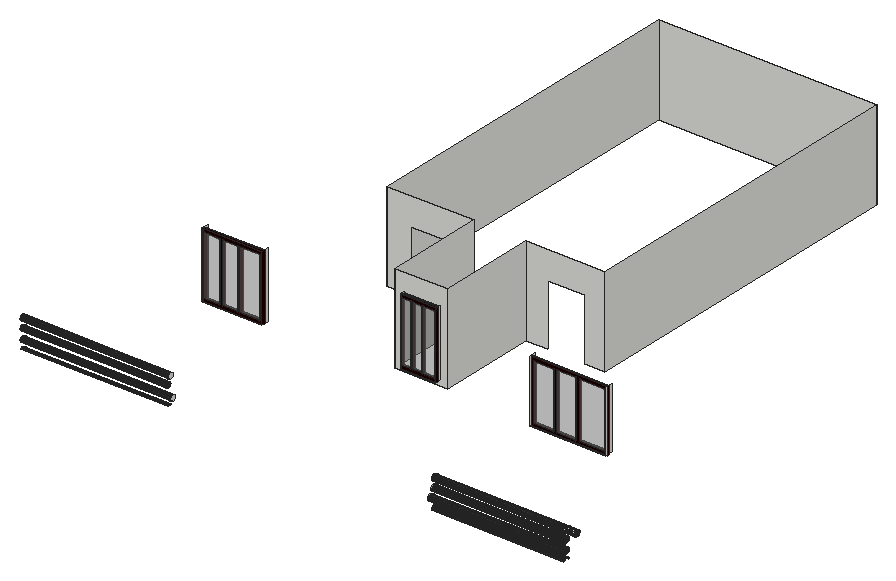
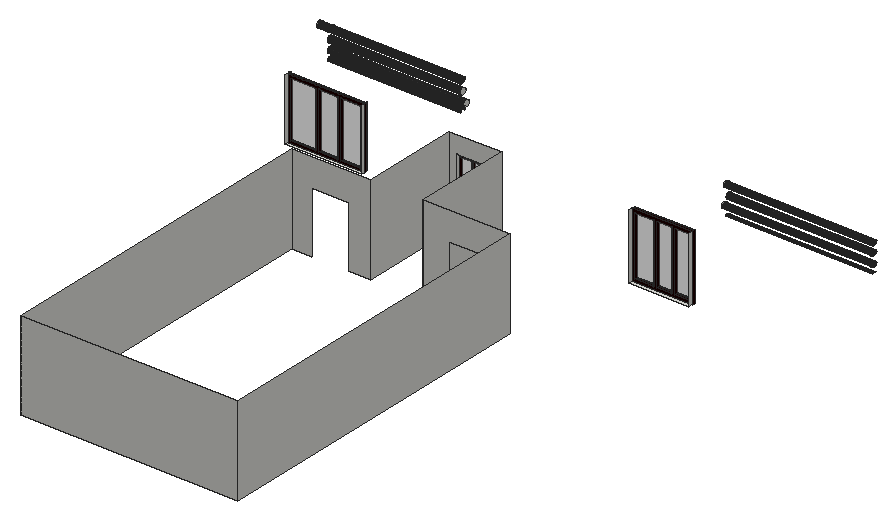
# SketchUp Ruby script. Lengths in inches.
U = 1.inch
M = Sketchup.active_model
def pt(a) = Geom::Point3d.new(a.map { |v| v * U })
def face(e, loops, mat)
  f = e.add_face(loops[0].map { |a| pt(a) })
  loops[1..].each { |l| e.add_face(l.map { |a| pt(a) }).erase! }
  f.material = f.back_material = mat if mat
  f
end
# faces: each face lists its corners as indices into pts; further lists are holes
def faces(e, pts, list, mat = nil) = list.each { |f| face(e, (f[0].is_a?(Array) ? f : [f]).map { |l| l.map { |i| pts[i] } }, mat) }
# xy, xz, yz: faces in a plane at the given z, y or x. An outline is a flat list of corners, or four numbers for a rectangle; further outlines are holes
def ring(l) = l.size == 4 ? [[l[0], l[1]], [l[2], l[1]], [l[2], l[3]], [l[0], l[3]]] : l.each_slice(2).to_a
def flat(e, list, mat, &to3) = list.each { |f| face(e, (f[0].is_a?(Array) ? f : [f]).map { |l| ring(l).map { |u, v| to3.(u, v) } }, mat) }
def xy(e, z, list, mat = nil) = flat(e, list, mat) { |x, y| [x, y, z] }
def xz(e, y, list, mat = nil) = flat(e, list, mat) { |x, z| [x, y, z] }
def yz(e, x, list, mat = nil) = flat(e, list, mat) { |y, z| [x, y, z] }
def lines(e, pts, list) = list.each { |a, b| e.add_line(pt(pts[a]), pt(pts[b])) }
# prism: a flat outline (further loops are holes) pulled along v
def prism(e, loops, v, mat = nil)
  f = face(e, loops, mat); d = Geom::Vector3d.new(v.map { |x| x * U })
  f.pushpull(f.normal.samedirection?(d) ? d.length : -d.length)
end
def box(e, o, s, mat = nil) = prism(e, [[o, [o[0] + s[0], o[1], o[2]], [o[0] + s[0], o[1] + s[1], o[2]], [o[0], o[1] + s[1], o[2]]]], [0, 0, s[2]], mat)
def at(x, y, z, deg = 0) = Geom::Transformation.translation(pt([x, y, z])) * Geom::Transformation.rotation(ORIGIN, Z_AXIS, deg.degrees)
def axes(o, x, y, z) = Geom::Transformation.new([*x, 0, *y, 0, *z, 0, *pt(o).to_a, 1])
def part(name) = M.definitions.add(name)
# library, detail: a bought-in or finely detailed component or shape, given as its bounding box
def library(name, o, s) = part(name).tap { |d| box(d.entities, o, s) }
def detail(e, o, s) = box(e.add_group.entities, o, s)
def put(e, d, t, mat = nil) = e.add_instance(d, t).tap { |i| i.material = mat if mat }
def group(e, t, mat = nil) = e.add_group.tap { |g| g.transformation = t; g.material = mat if mat }.entities
root = M.entities
M.materials.add("[Color A08]").color = [30, 0, 0]
M.materials.add("[Color M07]").color = [58, 58, 58]
M.materials.add("[Translucent Glass Gray]").color = [128, 128, 128]
M.materials["[Translucent Glass Gray]"].alpha = 0.5
c1 = part("Group\#2")
xy(c1.entities,0,[[0,0,95.3125,6]])
xy(c1.entities,4.01,[[4.01,0,28.72,6],[32.91,0,56.47,6],[60.66,0,91.31,6]],"[Color A08]")
xy(c1.entities,82.62,[[4.01,0,28.72,6],[32.91,0,56.47,6],[60.66,0,91.31,6]])
xy(c1.entities,86.625,[[0,0,95.3125,6]],"[Color A08]")
xz(c1.entities,0,[[[0,0,95.3125,86.625],[60.66,4.01,91.31,82.62],[4.01,4.01,28.72,82.62],[32.91,4.01,56.47,82.62]]],"[Color A08]")
xz(c1.entities,0,[[4.01,4.01,28.72,82.62],[32.91,4.01,56.47,82.62],[60.66,4.01,91.31,82.62]],"[Translucent Glass Gray]")
xz(c1.entities,6,[[[0,0,95.3125,86.625],[60.66,4.01,91.31,82.62],[4.01,4.01,28.72,82.62],[32.91,4.01,56.47,82.62]]],"[Color A08]")
yz(c1.entities,0,[[0,0,6,86.625]],"[Color A08]")
yz(c1.entities,4.01,[[0,4.01,6,82.62]],"[Color A08]")
yz(c1.entities,28.72,[[0,4.01,6,82.62]],"[Color A08]")
yz(c1.entities,32.91,[[0,4.01,6,82.62]],"[Color A08]")
yz(c1.entities,56.47,[[0,4.01,6,82.62]],"[Color A08]")
yz(c1.entities,60.66,[[0,4.01,6,82.62]],"[Color A08]")
yz(c1.entities,91.31,[[0,4.01,6,82.62]],"[Color A08]")
yz(c1.entities,95.3125,[[0,0,6,86.625]],"[Color A08]")
xy(root,88.1,[[362.91,203.5,408.97,209.5625]])
xy(root,90.39,[[124.03,183.0625,201.03,192.0625]])
xy(root,95.4,[[545.68,183.0625,644.56,192.0625]])
xz(root,209.5625,[[[351.23,81.5625,418.5,196.875],[362.91,88.1,408.97,174.47]]])
xz(root,336.0625,[[239.625,81.5625,239.625,196.875,351.23,196.875,351.23,81.5625,317.59,81.5625,317.59,160.875,269.59,160.875,269.59,81.5625],[418.5,81.5625,418.5,196.875,519.875,196.875,519.875,81.5625,494.24,81.5625,494.24,160.875,446.24,160.875,446.24,81.5625]])
xz(root,774.0625,[[239.625,81.5625,519.875,196.875]])
yz(root,124.03,[[183.0625,90.39,192.0625,175.07]])
yz(root,201.03,[[183.0625,90.39,192.0625,175.07]])
yz(root,223.46,[[8.45,113.18,9.29,113.3,10.08,113.62,10.75,114.14,11.27,114.81,11.59,115.59,11.7,116.43,11.59,117.28,11.27,118.06,10.75,118.73,10.08,119.25,9.29,119.57,8.45,119.68,7.61,119.57,6.83,119.25,6.15,118.73,5.64,118.06,5.3125,117.28,5.2,116.43,5.3125,115.59,5.64,114.81,6.15,114.14,6.83,113.62,7.61,113.3]])
yz(root,225.84,[[8.45,88,9.29,88.11,10.08,88.43,10.75,88.95,11.27,89.62,11.59,90.41,11.7,91.25,11.59,92.09,11.27,92.87,10.75,93.55,10.08,94.0625,9.29,94.39,8.45,94.5,7.61,94.39,6.83,94.0625,6.15,93.55,5.64,92.87,5.3125,92.09,5.2,91.25,5.3125,90.41,5.64,89.62,6.15,88.95,6.83,88.43,7.61,88.11]])
yz(root,239.625,[[336.0625,81.5625,774.0625,196.875]])
yz(root,351.23,[[209.5625,81.5625,336.0625,196.875]])
yz(root,362.91,[[203.5,88.1,209.5625,174.47]])
yz(root,408.97,[[203.5,88.1,209.5625,174.47]])
yz(root,418.5,[[209.5625,81.5625,336.0625,196.875]])
yz(root,519.875,[[336.0625,81.5625,774.0625,196.875]])
yz(root,545.68,[[183.0625,95.4,192.0625,174.78]])
yz(root,556.7,[[8.57,89.23,7.61,89.46,6.73,89.93,6.01,90.61,5.48,91.46,5.2,92.41,5.17,93.41,5.4,94.375,5.875,95.25,6.56,95.97,7.4,96.5,8.36,96.78,9.35,96.8125,10.32,96.58,11.2,96.11,11.92,95.42,12.44,94.58,12.73,93.625,12.76,92.63,12.53,91.66,12.05,90.79,11.37,90.0625,10.52,89.54,9.57,89.25]])
yz(root,561.08,[[8.57,101.66,7.61,101.89,6.73,102.37,6.01,103.05,5.48,103.9,5.2,104.85,5.17,105.84,5.4,106.8125,5.875,107.6875,6.56,108.41,7.4,108.93,8.36,109.22,9.35,109.25,10.32,109.02,11.2,108.55,11.92,107.86,12.44,107.02,12.73,106.0625,12.76,105.07,12.53,104.1,12.05,103.22,11.37,102.5,10.52,101.98,9.57,101.69]])
yz(root,644.56,[[183.0625,95.4,192.0625,174.78]])
p = [[31.52,6.83,82.0625],[31.52,6.15,81.55],[221.4,6.15,81.55],[221.4,6.83,82.0625],[31.52,10.75,81.55],[31.52,10.08,82.0625],
  [221.4,10.08,82.0625],[221.4,10.75,81.55],[732.77,5.17,81.78],[732.77,5.4,82.75],[561.7,5.4,82.75],[561.7,5.17,81.78],
  [732.77,12.44,82.95],[732.77,12.73,82],[561.7,12.73,82],[561.7,12.44,82.95],[31.52,7.61,82.39],[221.4,7.61,82.39],
  [31.52,9.29,82.39],[221.4,9.29,82.39],[31.52,8.45,82.5],[221.4,8.45,82.5],[732.77,5.875,83.625],[561.7,5.875,83.625],
  [732.77,11.92,83.8],[561.7,11.92,83.8],[732.77,6.56,84.35],[561.7,6.56,84.35],[732.77,11.2,84.48],[561.7,11.2,84.48],
  [732.77,7.4,84.87],[561.7,7.4,84.87],[732.77,10.32,84.96],[561.7,10.32,84.96],[732.77,8.36,85.16],[561.7,8.36,85.16],
  [732.77,9.35,85.1875],[561.7,9.35,85.1875],[31.52,7.61,88.11],[31.52,8.45,88],[225.84,8.45,88],[225.84,7.61,88.11],
  [31.52,9.29,88.11],[225.84,9.29,88.11],[31.52,6.83,88.43],[225.84,6.83,88.43],[31.52,10.08,88.43],[225.84,10.08,88.43],
  [31.52,6.15,88.95],[225.84,6.15,88.95],[31.52,10.75,88.95],[225.84,10.75,88.95],[31.52,5.64,89.62],[225.84,5.64,89.62],
  [31.52,11.27,89.62],[225.84,11.27,89.62],[732.77,8.57,89.23],[732.77,7.61,89.46],[556.7,7.61,89.46],[556.7,8.57,89.23],
  [732.77,9.57,89.25],[556.7,9.57,89.25],[732.77,10.52,89.54],[556.7,10.52,89.54],[732.77,6.73,89.93],[556.7,6.73,89.93],
  [732.77,11.37,90.0625],[556.7,11.37,90.0625],[31.52,5.3125,90.41],[225.84,5.3125,90.41],[31.52,11.59,90.41],[225.84,11.59,90.41],
  [732.77,6.01,90.61],[556.7,6.01,90.61],[732.77,12.05,90.79],[556.7,12.05,90.79],[31.52,5.2,91.25],[225.84,5.2,91.25],
  [31.52,11.7,91.25],[225.84,11.7,91.25],[732.77,5.48,91.46],[556.7,5.48,91.46],[732.77,12.53,91.66],[556.7,12.53,91.66],
  [31.52,5.3125,92.09],[225.84,5.3125,92.09],[31.52,11.59,92.09],[225.84,11.59,92.09],[732.77,5.2,92.41],[556.7,5.2,92.41],
  [732.77,12.76,92.63],[556.7,12.76,92.63],[31.52,5.64,92.87],[225.84,5.64,92.87],[31.52,11.27,92.87],[225.84,11.27,92.87],
  [732.77,5.17,93.41],[556.7,5.17,93.41],[732.77,12.73,93.625],[556.7,12.73,93.625],[31.52,6.15,93.55],[225.84,6.15,93.55],
  [31.52,10.75,93.55],[225.84,10.75,93.55],[732.77,5.4,94.375],[556.7,5.4,94.375],[31.52,6.83,94.0625],[225.84,6.83,94.0625],
  [31.52,10.08,94.0625],[225.84,10.08,94.0625],[732.77,12.44,94.58],[556.7,12.44,94.58],[31.52,7.61,94.39],[225.84,7.61,94.39],
  [31.52,9.29,94.39],[225.84,9.29,94.39],[732.77,5.875,95.25],[556.7,5.875,95.25],[31.52,8.45,94.5],[225.84,8.45,94.5],
  [732.77,11.92,95.42],[556.7,11.92,95.42],[732.77,6.56,95.97],[556.7,6.56,95.97],[732.77,11.2,96.11],[556.7,11.2,96.11],
  [732.77,7.4,96.5],[556.7,7.4,96.5],[732.77,10.32,96.58],[556.7,10.32,96.58],[732.77,8.36,96.78],[556.7,8.36,96.78],
  [732.77,9.35,96.8125],[556.7,9.35,96.8125],[31.52,7.61,101.61],[31.52,8.45,101.5],[219.71,8.45,101.5],[219.71,7.61,101.61],
  [31.52,9.29,101.61],[219.71,9.29,101.61],[31.52,6.83,101.93],[219.71,6.83,101.93],[31.52,10.08,101.93],[219.71,10.08,101.93],
  [732.77,8.57,101.66],[732.77,7.61,101.89],[561.08,7.61,101.89],[561.08,8.57,101.66],[732.77,9.57,101.69],[561.08,9.57,101.69],
  [732.77,10.52,101.98],[561.08,10.52,101.98],[31.52,6.15,102.45],[219.71,6.15,102.45],[732.77,6.73,102.37],[561.08,6.73,102.37],
  [31.52,10.75,102.45],[219.71,10.75,102.45],[732.77,11.37,102.5],[561.08,11.37,102.5],[31.52,5.64,103.12],[219.71,5.64,103.12],
  [732.77,6.01,103.05],[561.08,6.01,103.05],[31.52,11.27,103.12],[219.71,11.27,103.12],[732.77,12.05,103.22],[561.08,12.05,103.22],
  [732.77,5.48,103.9],[561.08,5.48,103.9],[31.52,5.3125,103.91],[219.71,5.3125,103.91],[31.52,11.59,103.91],[219.71,11.59,103.91],
  [732.77,12.53,104.1],[561.08,12.53,104.1],[31.52,5.2,104.75],[219.71,5.2,104.75],[732.77,5.2,104.85],[561.08,5.2,104.85],
  [31.52,11.7,104.75],[219.71,11.7,104.75],[732.77,12.76,105.07],[561.08,12.76,105.07],[31.52,5.3125,105.59],[219.71,5.3125,105.59],
  [31.52,11.59,105.59],[219.71,11.59,105.59],[732.77,5.17,105.84],[561.08,5.17,105.84],[732.77,12.73,106.0625],[561.08,12.73,106.0625],
  [31.52,5.64,106.37],[219.71,5.64,106.37],[31.52,11.27,106.37],[219.71,11.27,106.37],[732.77,5.4,106.8125],[561.08,5.4,106.8125],
  [732.77,12.44,107.02],[561.08,12.44,107.02],[31.52,6.15,107.05],[219.71,6.15,107.05],[31.52,10.75,107.05],[219.71,10.75,107.05],
  [732.77,5.875,107.6875],[561.08,5.875,107.6875],[31.52,6.83,107.5625],[219.71,6.83,107.5625],[31.52,10.08,107.5625],[219.71,10.08,107.5625],
  [732.77,11.92,107.86],[561.08,11.92,107.86],[31.52,7.61,107.89],[219.71,7.61,107.89],[31.52,9.29,107.89],[219.71,9.29,107.89],
  [732.77,6.56,108.41],[561.08,6.56,108.41],[31.52,8.45,108],[219.71,8.45,108],[732.77,11.2,108.55],[561.08,11.2,108.55],
  [732.77,7.4,108.93],[561.08,7.4,108.93],[732.77,10.32,109.02],[561.08,10.32,109.02],[732.77,8.36,109.22],[561.08,8.36,109.22],
  [732.77,9.35,109.25],[561.08,9.35,109.25],[31.52,7.61,113.3],[31.52,8.45,113.18],[223.46,8.45,113.18],[223.46,7.61,113.3],
  [31.52,9.29,113.3],[223.46,9.29,113.3],[31.52,6.83,113.62],[223.46,6.83,113.62],[31.52,10.08,113.62],[223.46,10.08,113.62],
  [31.52,6.15,114.14],[223.46,6.15,114.14],[31.52,10.75,114.14],[223.46,10.75,114.14],[31.52,5.64,114.81],[223.46,5.64,114.81],
  [31.52,11.27,114.81],[223.46,11.27,114.81],[732.77,8.57,114.16],[732.77,7.61,114.39],[562.05,7.61,114.39],[562.05,8.57,114.16],
  [746.625,8.57,114.16],[746.625,7.61,114.39],[732.77,9.57,114.19],[562.05,9.57,114.19],[746.625,9.57,114.19],[732.77,10.52,114.48],
  [562.05,10.52,114.48],[746.625,10.52,114.48],[732.77,6.73,114.87],[562.05,6.73,114.87],[746.625,6.73,114.87],[732.77,11.37,115],
  [562.05,11.37,115],[746.625,11.37,115],[31.52,5.3125,115.59],[223.46,5.3125,115.59],[31.52,11.59,115.59],[223.46,11.59,115.59],
  [732.77,6.01,115.55],[562.05,6.01,115.55],[746.625,6.01,115.55],[732.77,12.05,115.72],[562.05,12.05,115.72],[746.625,12.05,115.72],
  [732.77,5.48,116.4],[562.05,5.48,116.4],[746.625,5.48,116.4],[31.52,5.2,116.43],[223.46,5.2,116.43],[31.52,11.7,116.43],
  [223.46,11.7,116.43],[732.77,12.53,116.6],[562.05,12.53,116.6],[746.625,12.53,116.6],[31.52,5.3125,117.28],[223.46,5.3125,117.28],
  [732.77,5.2,117.35],[562.05,5.2,117.35],[746.625,5.2,117.35],[31.52,11.59,117.28],[223.46,11.59,117.28],[732.77,12.76,117.57],
  [562.05,12.76,117.57],[746.625,12.76,117.57],[732.77,5.17,118.34],[562.05,5.17,118.34],[746.625,5.17,118.34],[31.52,5.64,118.06],
  [223.46,5.64,118.06],[31.52,11.27,118.06],[223.46,11.27,118.06],[732.77,12.73,118.5625],[562.05,12.73,118.5625],[746.625,12.73,118.5625],
  [31.52,6.15,118.73],[223.46,6.15,118.73],[31.52,10.75,118.73],[223.46,10.75,118.73],[732.77,5.4,119.3125],[562.05,5.4,119.3125],
  [746.625,5.4,119.3125],[732.77,12.44,119.52],[562.05,12.44,119.52],[746.625,12.44,119.52],[31.52,6.83,119.25],[223.46,6.83,119.25],
  [31.52,10.08,119.25],[223.46,10.08,119.25],[31.52,7.61,119.57],[223.46,7.61,119.57],[31.52,9.29,119.57],[223.46,9.29,119.57],
  [732.77,5.875,120.1875],[562.05,5.875,120.1875],[746.625,5.875,120.1875],[732.77,11.92,120.36],[562.05,11.92,120.36],[746.625,11.92,120.36],
  [31.52,8.45,119.68],[223.46,8.45,119.68],[732.77,6.56,120.91],[562.05,6.56,120.91],[746.625,6.56,120.91],[732.77,11.2,121.05],
  [562.05,11.2,121.05],[746.625,11.2,121.05],[732.77,7.4,121.43],[562.05,7.4,121.43],[746.625,7.4,121.43],[732.77,10.32,121.52],
  [562.05,10.32,121.52],[746.625,10.32,121.52],[732.77,8.36,121.72],[562.05,8.36,121.72],[746.625,8.36,121.72],[732.77,9.35,121.75],
  [562.05,9.35,121.75],[746.625,9.35,121.75]]
faces(root,p,[[0,1,2,3],[4,5,6,7],[8,9,10,11],[12,13,14,15],[16,0,3,17],[5,18,19,6],[20,16,17,21],[18,20,21,19],
  [9,22,23,10],[24,12,15,25],[22,26,27,23],[28,24,25,29],[26,30,31,27],[32,28,29,33],[30,34,35,31],[36,32,33,37],
  [34,36,37,35],[38,39,40,41],[39,42,43,40],[44,38,41,45],[42,46,47,43],[48,44,45,49],[46,50,51,47],[52,48,49,53],
  [50,54,55,51],[56,57,58,59],[60,56,59,61],[62,60,61,63],[57,64,65,58],[66,62,63,67],[68,52,53,69],[54,70,71,55],
  [64,72,73,65],[74,66,67,75],[76,68,69,77],[70,78,79,71],[72,80,81,73],[82,74,75,83],[84,76,77,85],[78,86,87,79],
  [80,88,89,81],[90,82,83,91],[92,84,85,93],[86,94,95,87],[88,96,97,89],[98,90,91,99],[100,92,93,101],[94,102,103,95],
  [96,104,105,97],[106,100,101,107],[102,108,109,103],[110,98,99,111],[112,106,107,113],[108,114,115,109],[104,116,117,105],[118,112,113,119],
  [114,118,119,115],[120,110,111,121],[116,122,123,117],[124,120,121,125],[122,126,127,123],[128,124,125,129],[126,130,131,127],[132,128,129,133],
  [130,132,133,131],[134,135,136,137],[135,138,139,136],[140,134,137,141],[138,142,143,139],[144,145,146,147],[148,144,147,149],[150,148,149,151],
  [152,140,141,153],[145,154,155,146],[142,156,157,143],[158,150,151,159],[160,152,153,161],[154,162,163,155],[156,164,165,157],[166,158,159,167],
  [162,168,169,163],[170,160,161,171],[164,172,173,165],[174,166,167,175],[176,170,171,177],[168,178,179,169],[172,180,181,173],[182,174,175,183],
  [184,176,177,185],[180,186,187,181],[178,188,189,179],[190,182,183,191],[192,184,185,193],[186,194,195,187],[188,196,197,189],[198,190,191,199],
  [200,192,193,201],[194,202,203,195],[196,204,205,197],[206,200,201,207],[202,208,209,203],[210,198,199,211],[212,206,207,213],[208,214,215,209],
  [204,216,217,205],[218,212,213,219],[214,218,219,215],[220,210,211,221],[216,222,223,217],[224,220,221,225],[222,226,227,223],[228,224,225,229],
  [226,228,229,227],[230,231,232,233],[231,234,235,232],[236,230,233,237],[234,238,239,235],[240,236,237,241],[238,242,243,239],[244,240,241,245],
  [242,246,247,243],[248,249,250,251],[254,248,251,255],[257,254,255,258],[249,260,261,250],[263,257,258,264],[266,244,245,267],[246,268,269,247],
  [260,270,271,261],[273,263,264,274],[270,276,277,271],[279,266,267,280],[268,281,282,269],[283,273,274,284],[286,279,280,287],[276,288,289,277],
  [281,291,292,282],[293,283,284,294],[288,296,297,289],[299,286,287,300],[291,301,302,292],[303,293,294,304],[306,299,300,307],[301,308,309,302],
  [296,310,311,297],[313,303,304,314],[316,306,307,317],[308,318,319,309],[320,316,317,321],[318,322,323,319],[310,324,325,311],[327,313,314,328],
  [330,320,321,331],[322,330,331,323],[324,332,333,325],[335,327,328,336],[332,338,339,333],[341,335,336,342],[338,344,345,339],[347,341,342,348],
  [344,347,348,345]],"[Color M07]")
faces(root,p,[[249,248,252,253],[248,254,256,252],[254,257,259,256],[260,249,253,262],[257,263,265,259],[270,260,262,272],[263,273,275,265],[276,270,272,278],
  [273,283,285,275],[288,276,278,290],[283,293,295,285],[296,288,290,298],[293,303,305,295],[310,296,298,312],[303,313,315,305],[324,310,312,326],
  [313,327,329,315],[332,324,326,334],[327,335,337,329],[338,332,334,340],[335,341,343,337],[344,338,340,346],[341,347,349,343],[347,344,346,349]])
put(root,c1,axes([362.89,203.6,88.1],[0.48351,0,0],[0,0.43585,0],[0,0,0.99711]))
put(root,c1,axes([122.96,183.0625,90.39],[0.81915,0,0],[0,0.645,0],[0,0,0.97763]))
put(root,c1,axes([545.68,184.64,94.25],[1.04266,0,0],[0,0.4473,0],[0,0,0.92954]))
